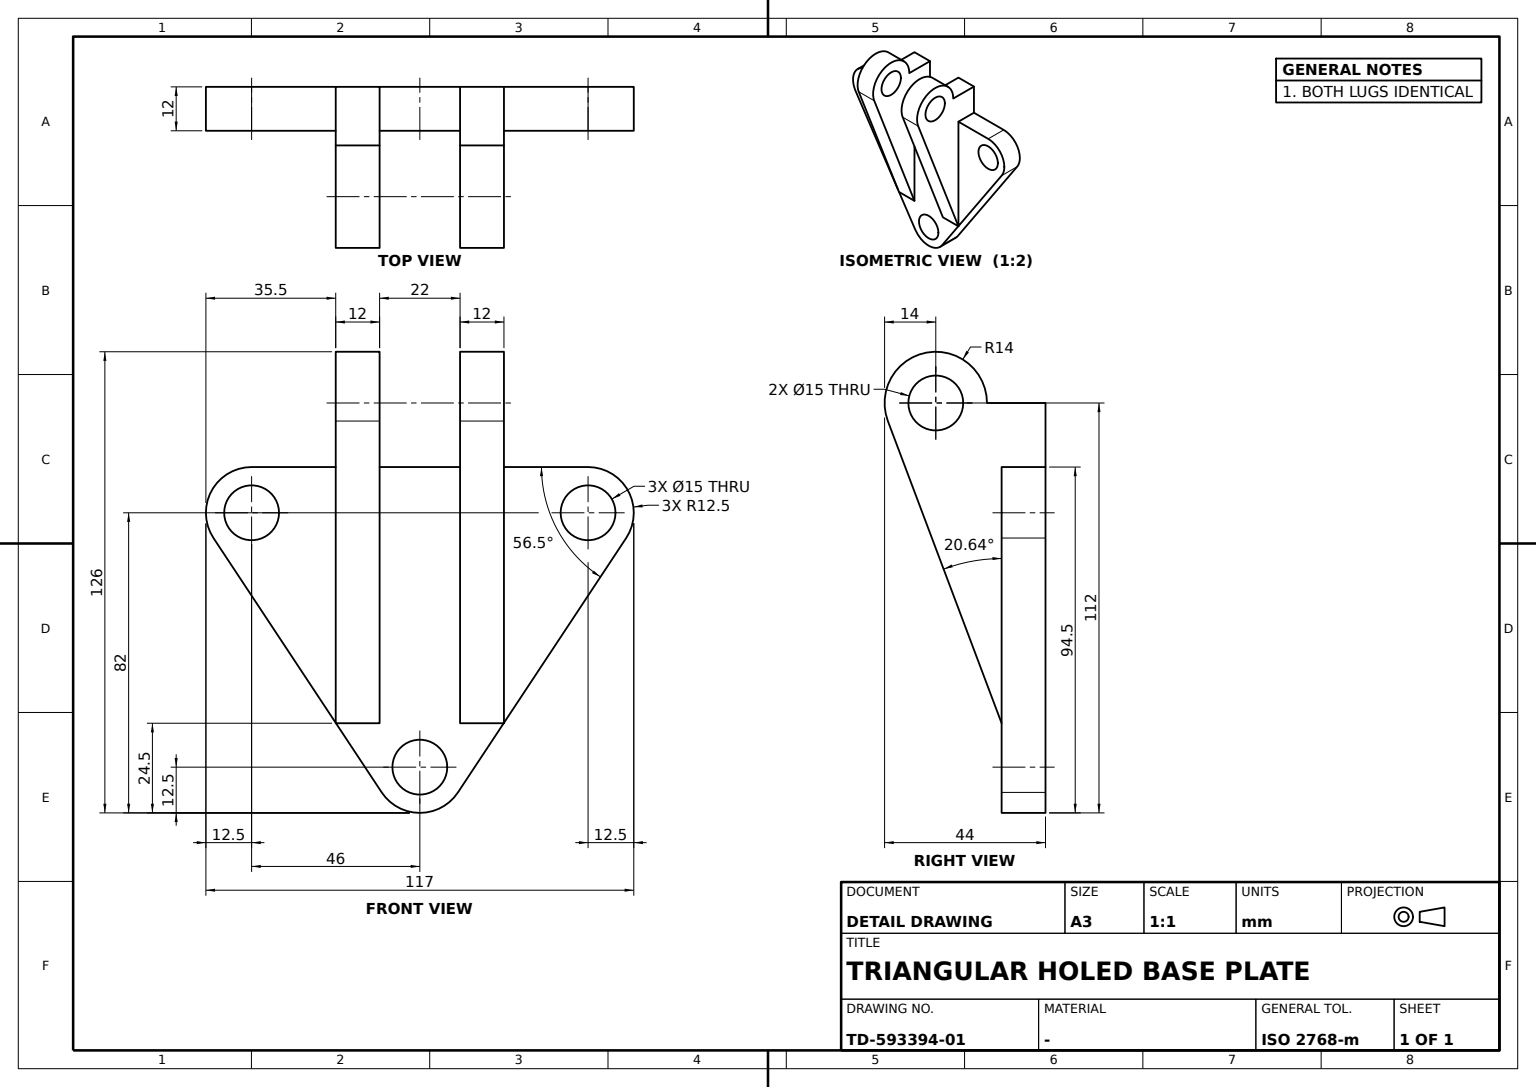
ISO-10303-21;
HEADER;
FILE_DESCRIPTION((''),'2;1');
FILE_NAME('','',(''),(''),'','','');
FILE_SCHEMA(('AUTOMOTIVE_DESIGN'));
ENDSEC;
DATA;
#1=APPLICATION_CONTEXT('');
#2=PRODUCT_CONTEXT('',#1,'mechanical');
#3=PRODUCT('','','',(#2));
#4=PRODUCT_DEFINITION_FORMATION('','',#3);
#5=PRODUCT_DEFINITION_CONTEXT('',#1,'design');
#6=PRODUCT_DEFINITION('','',#4,#5);
#7=PRODUCT_DEFINITION_SHAPE('','',#6);
#8=(LENGTH_UNIT()NAMED_UNIT(*)SI_UNIT(.MILLI.,.METRE.));
#9=(NAMED_UNIT(*)PLANE_ANGLE_UNIT()SI_UNIT($,.RADIAN.));
#10=(NAMED_UNIT(*)SI_UNIT($,.STERADIAN.)SOLID_ANGLE_UNIT());
#11=UNCERTAINTY_MEASURE_WITH_UNIT(LENGTH_MEASURE(1.E-05),#8,'distance_accuracy_value','');
#12=(GEOMETRIC_REPRESENTATION_CONTEXT(3)GLOBAL_UNCERTAINTY_ASSIGNED_CONTEXT((#11))GLOBAL_UNIT_ASSIGNED_CONTEXT((#8,#9,#10))REPRESENTATION_CONTEXT('',''));
#13=CARTESIAN_POINT('',(37.5,-11.,30.));
#14=VERTEX_POINT('',#13);
#15=CARTESIAN_POINT('',(22.5,-11.,30.));
#16=VERTEX_POINT('',#15);
#17=CARTESIAN_POINT('',(30.,-11.,30.));
#18=DIRECTION('',(0.,1.,0.));
#19=DIRECTION('',(-1.,0.,0.));
#20=AXIS2_PLACEMENT_3D('',#17,#18,#19);
#21=CIRCLE('',#20,7.5);
#22=EDGE_CURVE('',#14,#16,#21,.T.);
#23=ORIENTED_EDGE('',*,*,#22,.F.);
#24=EDGE_CURVE('',#16,#14,#21,.T.);
#25=ORIENTED_EDGE('',*,*,#24,.F.);
#26=EDGE_LOOP('',(#23,#25));
#27=FACE_BOUND('',#26,.T.);
#28=CARTESIAN_POINT('',(12.,-11.,12.5));
#29=VERTEX_POINT('',#28);
#30=CARTESIAN_POINT('',(0.,-11.,12.5));
#31=VERTEX_POINT('',#30);
#32=CARTESIAN_POINT('',(6.,-11.,12.5));
#33=VECTOR('',#19,1000.);
#34=LINE('',#32,#33);
#35=EDGE_CURVE('',#29,#31,#34,.T.);
#36=ORIENTED_EDGE('',*,*,#35,.T.);
#37=CARTESIAN_POINT('',(0.,-11.,30.));
#38=VERTEX_POINT('',#37);
#39=CARTESIAN_POINT('',(0.,-11.,21.25));
#40=DIRECTION('',(0.,0.,1.));
#41=VECTOR('',#40,1000.);
#42=LINE('',#39,#41);
#43=EDGE_CURVE('',#31,#38,#42,.T.);
#44=ORIENTED_EDGE('',*,*,#43,.T.);
#45=CARTESIAN_POINT('',(16.,-11.,30.));
#46=VERTEX_POINT('',#45);
#47=CARTESIAN_POINT('',(8.,-11.,30.));
#48=DIRECTION('',(1.,0.,0.));
#49=VECTOR('',#48,1000.);
#50=LINE('',#47,#49);
#51=EDGE_CURVE('',#38,#46,#50,.T.);
#52=ORIENTED_EDGE('',*,*,#51,.T.);
#53=CARTESIAN_POINT('',(43.101317,-11.,25.064872));
#54=VERTEX_POINT('',#53);
#55=CIRCLE('',#20,14.);
#56=EDGE_CURVE('',#46,#54,#55,.T.);
#57=ORIENTED_EDGE('',*,*,#56,.T.);
#58=CARTESIAN_POINT('',(12.,-11.,-57.5));
#59=VERTEX_POINT('',#58);
#60=CARTESIAN_POINT('',(27.550659,-11.,-16.217564));
#61=DIRECTION('',(-0.35250915,0.,-0.935808367));
#62=VECTOR('',#61,1000.);
#63=LINE('',#60,#62);
#64=EDGE_CURVE('',#54,#59,#63,.T.);
#65=ORIENTED_EDGE('',*,*,#64,.T.);
#66=CARTESIAN_POINT('',(12.,-11.,-22.5));
#67=LINE('',#66,#41);
#68=EDGE_CURVE('',#59,#29,#67,.T.);
#69=ORIENTED_EDGE('',*,*,#68,.T.);
#70=EDGE_LOOP('',(#36,#44,#52,#57,#65,#69));
#71=FACE_OUTER_BOUND('',#70,.T.);
#72=CARTESIAN_POINT('',(0.,-11.,0.));
#73=AXIS2_PLACEMENT_3D('',#72,#18,#19);
#74=PLANE('',#73);
#75=ADVANCED_FACE('',(#27,#71),#74,.T.);
#76=CARTESIAN_POINT('',(0.,38.5,0.));
#77=VERTEX_POINT('',#76);
#78=CARTESIAN_POINT('',(0.,53.5,0.));
#79=VERTEX_POINT('',#78);
#80=CARTESIAN_POINT('',(0.,46.,0.));
#81=AXIS2_PLACEMENT_3D('',#80,#48,#18);
#82=CIRCLE('',#81,7.5);
#83=EDGE_CURVE('',#77,#79,#82,.T.);
#84=ORIENTED_EDGE('',*,*,#83,.F.);
#85=CARTESIAN_POINT('',(12.,38.5,0.));
#86=VERTEX_POINT('',#85);
#87=CARTESIAN_POINT('',(6.,38.5,0.));
#88=LINE('',#87,#49);
#89=EDGE_CURVE('',#77,#86,#88,.T.);
#90=ORIENTED_EDGE('',*,*,#89,.T.);
#91=CARTESIAN_POINT('',(12.,53.5,0.));
#92=VERTEX_POINT('',#91);
#93=CARTESIAN_POINT('',(12.,46.,0.));
#94=AXIS2_PLACEMENT_3D('',#93,#48,#18);
#95=CIRCLE('',#94,7.5);
#96=EDGE_CURVE('',#86,#92,#95,.T.);
#97=ORIENTED_EDGE('',*,*,#96,.T.);
#98=CARTESIAN_POINT('',(6.,53.5,0.));
#99=LINE('',#98,#49);
#100=EDGE_CURVE('',#79,#92,#99,.T.);
#101=ORIENTED_EDGE('',*,*,#100,.F.);
#102=EDGE_LOOP('',(#84,#90,#97,#101));
#103=FACE_OUTER_BOUND('',#102,.T.);
#104=CARTESIAN_POINT('',(6.,46.,0.));
#105=AXIS2_PLACEMENT_3D('',#104,#19,#18);
#106=CYLINDRICAL_SURFACE('',#105,7.5);
#107=ADVANCED_FACE('',(#103),#106,.F.);
#108=CARTESIAN_POINT('',(0.,11.,30.));
#109=VERTEX_POINT('',#108);
#110=CARTESIAN_POINT('',(16.,11.,30.));
#111=VERTEX_POINT('',#110);
#112=CARTESIAN_POINT('',(8.,11.,30.));
#113=LINE('',#112,#49);
#114=EDGE_CURVE('',#109,#111,#113,.T.);
#115=ORIENTED_EDGE('',*,*,#114,.T.);
#116=CARTESIAN_POINT('',(16.,23.,30.));
#117=VERTEX_POINT('',#116);
#118=CARTESIAN_POINT('',(16.,17.,30.));
#119=VECTOR('',#18,1000.);
#120=LINE('',#118,#119);
#121=EDGE_CURVE('',#111,#117,#120,.T.);
#122=ORIENTED_EDGE('',*,*,#121,.T.);
#123=CARTESIAN_POINT('',(0.,23.,30.));
#124=VERTEX_POINT('',#123);
#125=CARTESIAN_POINT('',(8.,23.,30.));
#126=LINE('',#125,#49);
#127=EDGE_CURVE('',#124,#117,#126,.T.);
#128=ORIENTED_EDGE('',*,*,#127,.F.);
#129=CARTESIAN_POINT('',(0.,17.,30.));
#130=LINE('',#129,#119);
#131=EDGE_CURVE('',#109,#124,#130,.T.);
#132=ORIENTED_EDGE('',*,*,#131,.F.);
#133=EDGE_LOOP('',(#115,#122,#128,#132));
#134=FACE_OUTER_BOUND('',#133,.T.);
#135=CARTESIAN_POINT('',(16.,0.,30.));
#136=DIRECTION('',(0.,0.,-1.));
#137=AXIS2_PLACEMENT_3D('',#135,#136,#19);
#138=PLANE('',#137);
#139=ADVANCED_FACE('',(#134),#138,.F.);
#140=CARTESIAN_POINT('',(0.,-7.5,-69.5));
#141=VERTEX_POINT('',#140);
#142=CARTESIAN_POINT('',(12.,-7.5,-69.5));
#143=VERTEX_POINT('',#142);
#144=CARTESIAN_POINT('',(6.,-7.5,-69.5));
#145=LINE('',#144,#49);
#146=EDGE_CURVE('',#141,#143,#145,.T.);
#147=ORIENTED_EDGE('',*,*,#146,.F.);
#148=CARTESIAN_POINT('',(0.,7.5,-69.5));
#149=VERTEX_POINT('',#148);
#150=CARTESIAN_POINT('',(0.,0.,-69.5));
#151=AXIS2_PLACEMENT_3D('',#150,#48,#18);
#152=CIRCLE('',#151,7.5);
#153=EDGE_CURVE('',#149,#141,#152,.T.);
#154=ORIENTED_EDGE('',*,*,#153,.F.);
#155=CARTESIAN_POINT('',(12.,7.5,-69.5));
#156=VERTEX_POINT('',#155);
#157=CARTESIAN_POINT('',(6.,7.5,-69.5));
#158=LINE('',#157,#49);
#159=EDGE_CURVE('',#149,#156,#158,.T.);
#160=ORIENTED_EDGE('',*,*,#159,.T.);
#161=CARTESIAN_POINT('',(12.,0.,-69.5));
#162=AXIS2_PLACEMENT_3D('',#161,#48,#18);
#163=CIRCLE('',#162,7.5);
#164=EDGE_CURVE('',#156,#143,#163,.T.);
#165=ORIENTED_EDGE('',*,*,#164,.T.);
#166=EDGE_LOOP('',(#147,#154,#160,#165));
#167=FACE_OUTER_BOUND('',#166,.T.);
#168=CARTESIAN_POINT('',(6.,0.,-69.5));
#169=AXIS2_PLACEMENT_3D('',#168,#19,#18);
#170=CYLINDRICAL_SURFACE('',#169,7.5);
#171=ADVANCED_FACE('',(#167),#170,.F.);
#172=CARTESIAN_POINT('',(37.5,11.,30.));
#173=VERTEX_POINT('',#172);
#174=CARTESIAN_POINT('',(37.5,23.,30.));
#175=VERTEX_POINT('',#174);
#176=CARTESIAN_POINT('',(37.5,17.,30.));
#177=LINE('',#176,#119);
#178=EDGE_CURVE('',#173,#175,#177,.T.);
#179=ORIENTED_EDGE('',*,*,#178,.T.);
#180=CARTESIAN_POINT('',(22.5,23.,30.));
#181=VERTEX_POINT('',#180);
#182=CARTESIAN_POINT('',(30.,23.,30.));
#183=AXIS2_PLACEMENT_3D('',#182,#18,#19);
#184=CIRCLE('',#183,7.5);
#185=EDGE_CURVE('',#175,#181,#184,.T.);
#186=ORIENTED_EDGE('',*,*,#185,.T.);
#187=CARTESIAN_POINT('',(22.5,11.,30.));
#188=VERTEX_POINT('',#187);
#189=CARTESIAN_POINT('',(22.5,17.,30.));
#190=LINE('',#189,#119);
#191=EDGE_CURVE('',#188,#181,#190,.T.);
#192=ORIENTED_EDGE('',*,*,#191,.F.);
#193=CARTESIAN_POINT('',(30.,11.,30.));
#194=AXIS2_PLACEMENT_3D('',#193,#18,#19);
#195=CIRCLE('',#194,7.5);
#196=EDGE_CURVE('',#173,#188,#195,.T.);
#197=ORIENTED_EDGE('',*,*,#196,.F.);
#198=EDGE_LOOP('',(#179,#186,#192,#197));
#199=FACE_OUTER_BOUND('',#198,.T.);
#200=CARTESIAN_POINT('',(30.,17.,30.));
#201=DIRECTION('',(0.,-1.,0.));
#202=AXIS2_PLACEMENT_3D('',#200,#201,#19);
#203=CYLINDRICAL_SURFACE('',#202,7.5);
#204=ADVANCED_FACE('',(#199),#203,.F.);
#205=CARTESIAN_POINT('',(0.,11.,12.5));
#206=VERTEX_POINT('',#205);
#207=CARTESIAN_POINT('',(0.,0.,12.5));
#208=VECTOR('',#201,1000.);
#209=LINE('',#207,#208);
#210=EDGE_CURVE('',#206,#31,#209,.T.);
#211=ORIENTED_EDGE('',*,*,#210,.T.);
#212=ORIENTED_EDGE('',*,*,#35,.F.);
#213=CARTESIAN_POINT('',(12.,11.,12.5));
#214=VERTEX_POINT('',#213);
#215=CARTESIAN_POINT('',(12.,0.,12.5));
#216=LINE('',#215,#208);
#217=EDGE_CURVE('',#214,#29,#216,.T.);
#218=ORIENTED_EDGE('',*,*,#217,.F.);
#219=CARTESIAN_POINT('',(6.,11.,12.5));
#220=LINE('',#219,#33);
#221=EDGE_CURVE('',#214,#206,#220,.T.);
#222=ORIENTED_EDGE('',*,*,#221,.T.);
#223=EDGE_LOOP('',(#211,#212,#218,#222));
#224=FACE_OUTER_BOUND('',#223,.T.);
#225=CARTESIAN_POINT('',(0.,-46.,12.5));
#226=AXIS2_PLACEMENT_3D('',#225,#136,#18);
#227=PLANE('',#226);
#228=ADVANCED_FACE('',(#224),#227,.F.);
#229=CARTESIAN_POINT('',(12.,56.423645,-6.899103));
#230=VERTEX_POINT('',#229);
#231=CARTESIAN_POINT('',(12.,23.,-57.397871));
#232=VERTEX_POINT('',#231);
#233=CARTESIAN_POINT('',(12.,39.711823,-32.148487));
#234=DIRECTION('',(0.,-0.551928254,-0.833891601));
#235=VECTOR('',#234,1000.);
#236=LINE('',#233,#235);
#237=EDGE_CURVE('',#230,#232,#236,.T.);
#238=ORIENTED_EDGE('',*,*,#237,.T.);
#239=CARTESIAN_POINT('',(12.,22.932404,-57.5));
#240=VERTEX_POINT('',#239);
#241=CARTESIAN_POINT('',(12.,22.966202,-57.448936));
#242=LINE('',#241,#235);
#243=EDGE_CURVE('',#232,#240,#242,.T.);
#244=ORIENTED_EDGE('',*,*,#243,.T.);
#245=CARTESIAN_POINT('',(12.,10.423645,-76.399103));
#246=VERTEX_POINT('',#245);
#247=CARTESIAN_POINT('',(12.,16.678024,-66.949552));
#248=LINE('',#247,#235);
#249=EDGE_CURVE('',#240,#246,#248,.T.);
#250=ORIENTED_EDGE('',*,*,#249,.T.);
#251=CARTESIAN_POINT('',(0.,10.423645,-76.399103));
#252=VERTEX_POINT('',#251);
#253=CARTESIAN_POINT('',(6.,10.423645,-76.399103));
#254=LINE('',#253,#49);
#255=EDGE_CURVE('',#252,#246,#254,.T.);
#256=ORIENTED_EDGE('',*,*,#255,.F.);
#257=CARTESIAN_POINT('',(0.,56.423645,-6.899103));
#258=VERTEX_POINT('',#257);
#259=CARTESIAN_POINT('',(0.,33.423645,-41.649103));
#260=LINE('',#259,#235);
#261=EDGE_CURVE('',#258,#252,#260,.T.);
#262=ORIENTED_EDGE('',*,*,#261,.F.);
#263=CARTESIAN_POINT('',(6.,56.423645,-6.899103));
#264=LINE('',#263,#49);
#265=EDGE_CURVE('',#258,#230,#264,.T.);
#266=ORIENTED_EDGE('',*,*,#265,.T.);
#267=EDGE_LOOP('',(#238,#244,#250,#256,#262,#266));
#268=FACE_OUTER_BOUND('',#267,.T.);
#269=DIRECTION('',(0.,0.833891601,-0.551928254));
#270=DIRECTION('',(0.,0.551928254,0.833891601));
#271=AXIS2_PLACEMENT_3D('',#251,#269,#270);
#272=PLANE('',#271);
#273=ADVANCED_FACE('',(#268),#272,.T.);
#274=CARTESIAN_POINT('',(0.,58.5,0.));
#275=VERTEX_POINT('',#274);
#276=CIRCLE('',#81,12.5);
#277=EDGE_CURVE('',#258,#275,#276,.T.);
#278=ORIENTED_EDGE('',*,*,#277,.T.);
#279=CARTESIAN_POINT('',(12.,58.5,0.));
#280=VERTEX_POINT('',#279);
#281=CARTESIAN_POINT('',(6.,58.5,0.));
#282=LINE('',#281,#33);
#283=EDGE_CURVE('',#280,#275,#282,.T.);
#284=ORIENTED_EDGE('',*,*,#283,.F.);
#285=CIRCLE('',#94,12.5);
#286=EDGE_CURVE('',#230,#280,#285,.T.);
#287=ORIENTED_EDGE('',*,*,#286,.F.);
#288=ORIENTED_EDGE('',*,*,#265,.F.);
#289=EDGE_LOOP('',(#278,#284,#287,#288));
#290=FACE_OUTER_BOUND('',#289,.T.);
#291=CYLINDRICAL_SURFACE('',#105,12.5);
#292=ADVANCED_FACE('',(#290),#291,.T.);
#293=CARTESIAN_POINT('',(43.101317,-23.,25.064872));
#294=VERTEX_POINT('',#293);
#295=CARTESIAN_POINT('',(43.101317,17.,25.064872));
#296=LINE('',#295,#208);
#297=EDGE_CURVE('',#54,#294,#296,.T.);
#298=ORIENTED_EDGE('',*,*,#297,.F.);
#299=ORIENTED_EDGE('',*,*,#56,.F.);
#300=CARTESIAN_POINT('',(16.,-23.,30.));
#301=VERTEX_POINT('',#300);
#302=LINE('',#118,#208);
#303=EDGE_CURVE('',#46,#301,#302,.T.);
#304=ORIENTED_EDGE('',*,*,#303,.T.);
#305=CARTESIAN_POINT('',(30.,-23.,30.));
#306=AXIS2_PLACEMENT_3D('',#305,#18,#19);
#307=CIRCLE('',#306,14.);
#308=EDGE_CURVE('',#301,#294,#307,.T.);
#309=ORIENTED_EDGE('',*,*,#308,.T.);
#310=EDGE_LOOP('',(#298,#299,#304,#309));
#311=FACE_OUTER_BOUND('',#310,.T.);
#312=CYLINDRICAL_SURFACE('',#202,14.);
#313=ADVANCED_FACE('',(#311),#312,.T.);
#314=CARTESIAN_POINT('',(43.101317,23.,25.064872));
#315=VERTEX_POINT('',#314);
#316=CARTESIAN_POINT('',(12.,23.,-57.5));
#317=VERTEX_POINT('',#316);
#318=CARTESIAN_POINT('',(27.550659,23.,-16.217564));
#319=LINE('',#318,#62);
#320=EDGE_CURVE('',#315,#317,#319,.T.);
#321=ORIENTED_EDGE('',*,*,#320,.F.);
#322=CARTESIAN_POINT('',(43.101317,11.,25.064872));
#323=VERTEX_POINT('',#322);
#324=LINE('',#295,#119);
#325=EDGE_CURVE('',#323,#315,#324,.T.);
#326=ORIENTED_EDGE('',*,*,#325,.F.);
#327=CARTESIAN_POINT('',(12.,11.,-57.5));
#328=VERTEX_POINT('',#327);
#329=CARTESIAN_POINT('',(27.550659,11.,-16.217564));
#330=LINE('',#329,#62);
#331=EDGE_CURVE('',#323,#328,#330,.T.);
#332=ORIENTED_EDGE('',*,*,#331,.T.);
#333=CARTESIAN_POINT('',(12.,16.966202,-57.5));
#334=LINE('',#333,#119);
#335=EDGE_CURVE('',#328,#240,#334,.T.);
#336=ORIENTED_EDGE('',*,*,#335,.T.);
#337=CARTESIAN_POINT('',(12.,22.966202,-57.5));
#338=LINE('',#337,#119);
#339=EDGE_CURVE('',#240,#317,#338,.T.);
#340=ORIENTED_EDGE('',*,*,#339,.T.);
#341=EDGE_LOOP('',(#321,#326,#332,#336,#340));
#342=FACE_OUTER_BOUND('',#341,.T.);
#343=CARTESIAN_POINT('',(43.101317,0.,25.064872));
#344=DIRECTION('',(0.935808367,0.,-0.35250915));
#345=AXIS2_PLACEMENT_3D('',#343,#344,#61);
#346=PLANE('',#345);
#347=ADVANCED_FACE('',(#342),#346,.T.);
#348=EDGE_CURVE('',#92,#86,#95,.T.);
#349=ORIENTED_EDGE('',*,*,#348,.F.);
#350=ORIENTED_EDGE('',*,*,#96,.F.);
#351=EDGE_LOOP('',(#349,#350));
#352=FACE_BOUND('',#351,.T.);
#353=ORIENTED_EDGE('',*,*,#286,.T.);
#354=CARTESIAN_POINT('',(12.,46.,12.5));
#355=VERTEX_POINT('',#354);
#356=EDGE_CURVE('',#280,#355,#285,.T.);
#357=ORIENTED_EDGE('',*,*,#356,.T.);
#358=CARTESIAN_POINT('',(12.,23.,12.5));
#359=VERTEX_POINT('',#358);
#360=CARTESIAN_POINT('',(12.,34.5,12.5));
#361=LINE('',#360,#208);
#362=EDGE_CURVE('',#355,#359,#361,.T.);
#363=ORIENTED_EDGE('',*,*,#362,.T.);
#364=CARTESIAN_POINT('',(12.,23.,-22.448936));
#365=LINE('',#364,#41);
#366=EDGE_CURVE('',#232,#359,#365,.T.);
#367=ORIENTED_EDGE('',*,*,#366,.F.);
#368=ORIENTED_EDGE('',*,*,#237,.F.);
#369=EDGE_LOOP('',(#353,#357,#363,#367,#368));
#370=FACE_OUTER_BOUND('',#369,.T.);
#371=CARTESIAN_POINT('',(12.,0.,0.));
#372=AXIS2_PLACEMENT_3D('',#371,#48,#18);
#373=PLANE('',#372);
#374=ADVANCED_FACE('',(#352,#370),#373,.T.);
#375=CARTESIAN_POINT('',(0.,46.,12.5));
#376=VERTEX_POINT('',#375);
#377=CARTESIAN_POINT('',(0.,23.,12.5));
#378=VERTEX_POINT('',#377);
#379=CARTESIAN_POINT('',(0.,34.5,12.5));
#380=LINE('',#379,#208);
#381=EDGE_CURVE('',#376,#378,#380,.T.);
#382=ORIENTED_EDGE('',*,*,#381,.T.);
#383=CARTESIAN_POINT('',(6.,23.,12.5));
#384=LINE('',#383,#33);
#385=EDGE_CURVE('',#359,#378,#384,.T.);
#386=ORIENTED_EDGE('',*,*,#385,.F.);
#387=ORIENTED_EDGE('',*,*,#362,.F.);
#388=CARTESIAN_POINT('',(6.,46.,12.5));
#389=LINE('',#388,#49);
#390=EDGE_CURVE('',#376,#355,#389,.T.);
#391=ORIENTED_EDGE('',*,*,#390,.F.);
#392=EDGE_LOOP('',(#382,#386,#387,#391));
#393=FACE_OUTER_BOUND('',#392,.T.);
#394=ADVANCED_FACE('',(#393),#227,.F.);
#395=CARTESIAN_POINT('',(12.,23.,-57.448936));
#396=LINE('',#395,#41);
#397=EDGE_CURVE('',#317,#232,#396,.T.);
#398=ORIENTED_EDGE('',*,*,#397,.F.);
#399=ORIENTED_EDGE('',*,*,#339,.F.);
#400=ORIENTED_EDGE('',*,*,#243,.F.);
#401=EDGE_LOOP('',(#398,#399,#400));
#402=FACE_OUTER_BOUND('',#401,.T.);
#403=ADVANCED_FACE('',(#402),#373,.F.);
#404=CARTESIAN_POINT('',(0.,-38.5,0.));
#405=VERTEX_POINT('',#404);
#406=CARTESIAN_POINT('',(12.,-38.5,0.));
#407=VERTEX_POINT('',#406);
#408=CARTESIAN_POINT('',(6.,-38.5,0.));
#409=LINE('',#408,#49);
#410=EDGE_CURVE('',#405,#407,#409,.T.);
#411=ORIENTED_EDGE('',*,*,#410,.F.);
#412=CARTESIAN_POINT('',(0.,-53.5,0.));
#413=VERTEX_POINT('',#412);
#414=CARTESIAN_POINT('',(0.,-46.,0.));
#415=AXIS2_PLACEMENT_3D('',#414,#48,#18);
#416=CIRCLE('',#415,7.5);
#417=EDGE_CURVE('',#413,#405,#416,.T.);
#418=ORIENTED_EDGE('',*,*,#417,.F.);
#419=CARTESIAN_POINT('',(12.,-53.5,0.));
#420=VERTEX_POINT('',#419);
#421=CARTESIAN_POINT('',(6.,-53.5,0.));
#422=LINE('',#421,#49);
#423=EDGE_CURVE('',#413,#420,#422,.T.);
#424=ORIENTED_EDGE('',*,*,#423,.T.);
#425=CARTESIAN_POINT('',(12.,-46.,0.));
#426=AXIS2_PLACEMENT_3D('',#425,#48,#18);
#427=CIRCLE('',#426,7.5);
#428=EDGE_CURVE('',#420,#407,#427,.T.);
#429=ORIENTED_EDGE('',*,*,#428,.T.);
#430=EDGE_LOOP('',(#411,#418,#424,#429));
#431=FACE_OUTER_BOUND('',#430,.T.);
#432=CARTESIAN_POINT('',(6.,-46.,0.));
#433=AXIS2_PLACEMENT_3D('',#432,#19,#18);
#434=CYLINDRICAL_SURFACE('',#433,7.5);
#435=ADVANCED_FACE('',(#431),#434,.F.);
#436=ORIENTED_EDGE('',*,*,#114,.F.);
#437=CARTESIAN_POINT('',(0.,11.,21.25));
#438=LINE('',#437,#41);
#439=EDGE_CURVE('',#206,#109,#438,.T.);
#440=ORIENTED_EDGE('',*,*,#439,.F.);
#441=ORIENTED_EDGE('',*,*,#221,.F.);
#442=CARTESIAN_POINT('',(12.,11.,-22.5));
#443=LINE('',#442,#41);
#444=EDGE_CURVE('',#328,#214,#443,.T.);
#445=ORIENTED_EDGE('',*,*,#444,.F.);
#446=ORIENTED_EDGE('',*,*,#331,.F.);
#447=CIRCLE('',#194,14.);
#448=EDGE_CURVE('',#111,#323,#447,.T.);
#449=ORIENTED_EDGE('',*,*,#448,.F.);
#450=EDGE_LOOP('',(#436,#440,#441,#445,#446,#449));
#451=FACE_OUTER_BOUND('',#450,.T.);
#452=EDGE_CURVE('',#188,#173,#195,.T.);
#453=ORIENTED_EDGE('',*,*,#452,.T.);
#454=ORIENTED_EDGE('',*,*,#196,.T.);
#455=EDGE_LOOP('',(#453,#454));
#456=FACE_BOUND('',#455,.T.);
#457=CARTESIAN_POINT('',(0.,11.,0.));
#458=AXIS2_PLACEMENT_3D('',#457,#18,#19);
#459=PLANE('',#458);
#460=ADVANCED_FACE('',(#451,#456),#459,.F.);
#461=CARTESIAN_POINT('',(0.,-10.423645,-76.399103));
#462=VERTEX_POINT('',#461);
#463=CARTESIAN_POINT('',(12.,-10.423645,-76.399103));
#464=VERTEX_POINT('',#463);
#465=CARTESIAN_POINT('',(6.,-10.423645,-76.399103));
#466=LINE('',#465,#49);
#467=EDGE_CURVE('',#462,#464,#466,.T.);
#468=ORIENTED_EDGE('',*,*,#467,.F.);
#469=CIRCLE('',#151,12.5);
#470=EDGE_CURVE('',#462,#252,#469,.T.);
#471=ORIENTED_EDGE('',*,*,#470,.T.);
#472=ORIENTED_EDGE('',*,*,#255,.T.);
#473=CIRCLE('',#162,12.5);
#474=EDGE_CURVE('',#464,#246,#473,.T.);
#475=ORIENTED_EDGE('',*,*,#474,.F.);
#476=EDGE_LOOP('',(#468,#471,#472,#475));
#477=FACE_OUTER_BOUND('',#476,.T.);
#478=CYLINDRICAL_SURFACE('',#169,12.5);
#479=ADVANCED_FACE('',(#477),#478,.T.);
#480=ORIENTED_EDGE('',*,*,#83,.T.);
#481=EDGE_CURVE('',#79,#77,#82,.T.);
#482=ORIENTED_EDGE('',*,*,#481,.T.);
#483=EDGE_LOOP('',(#480,#482));
#484=FACE_BOUND('',#483,.T.);
#485=ORIENTED_EDGE('',*,*,#470,.F.);
#486=CARTESIAN_POINT('',(0.,-56.423645,-6.899103));
#487=VERTEX_POINT('',#486);
#488=CARTESIAN_POINT('',(0.,-33.423645,-41.649103));
#489=DIRECTION('',(0.,0.551928254,-0.833891601));
#490=VECTOR('',#489,1000.);
#491=LINE('',#488,#490);
#492=EDGE_CURVE('',#487,#462,#491,.T.);
#493=ORIENTED_EDGE('',*,*,#492,.F.);
#494=VERTEX_POINT('',#225);
#495=CIRCLE('',#415,12.5);
#496=EDGE_CURVE('',#494,#487,#495,.T.);
#497=ORIENTED_EDGE('',*,*,#496,.F.);
#498=CARTESIAN_POINT('',(0.,-23.,12.5));
#499=VERTEX_POINT('',#498);
#500=CARTESIAN_POINT('',(0.,-34.5,12.5));
#501=LINE('',#500,#208);
#502=EDGE_CURVE('',#499,#494,#501,.T.);
#503=ORIENTED_EDGE('',*,*,#502,.F.);
#504=CARTESIAN_POINT('',(0.,-23.,30.));
#505=VERTEX_POINT('',#504);
#506=CARTESIAN_POINT('',(0.,-23.,21.25));
#507=LINE('',#506,#41);
#508=EDGE_CURVE('',#499,#505,#507,.T.);
#509=ORIENTED_EDGE('',*,*,#508,.T.);
#510=CARTESIAN_POINT('',(0.,-17.,30.));
#511=LINE('',#510,#208);
#512=EDGE_CURVE('',#38,#505,#511,.T.);
#513=ORIENTED_EDGE('',*,*,#512,.F.);
#514=ORIENTED_EDGE('',*,*,#43,.F.);
#515=ORIENTED_EDGE('',*,*,#210,.F.);
#516=ORIENTED_EDGE('',*,*,#439,.T.);
#517=ORIENTED_EDGE('',*,*,#131,.T.);
#518=CARTESIAN_POINT('',(0.,23.,21.25));
#519=LINE('',#518,#41);
#520=EDGE_CURVE('',#378,#124,#519,.T.);
#521=ORIENTED_EDGE('',*,*,#520,.F.);
#522=ORIENTED_EDGE('',*,*,#381,.F.);
#523=EDGE_CURVE('',#275,#376,#276,.T.);
#524=ORIENTED_EDGE('',*,*,#523,.F.);
#525=ORIENTED_EDGE('',*,*,#277,.F.);
#526=ORIENTED_EDGE('',*,*,#261,.T.);
#527=EDGE_LOOP('',(#485,#493,#497,#503,#509,#513,#514,#515,#516,#517,#521,#522,#524,#525,#526));
#528=FACE_OUTER_BOUND('',#527,.T.);
#529=ORIENTED_EDGE('',*,*,#153,.T.);
#530=EDGE_CURVE('',#141,#149,#152,.T.);
#531=ORIENTED_EDGE('',*,*,#530,.T.);
#532=EDGE_LOOP('',(#529,#531));
#533=FACE_BOUND('',#532,.T.);
#534=EDGE_CURVE('',#405,#413,#416,.T.);
#535=ORIENTED_EDGE('',*,*,#534,.T.);
#536=ORIENTED_EDGE('',*,*,#417,.T.);
#537=EDGE_LOOP('',(#535,#536));
#538=FACE_BOUND('',#537,.T.);
#539=CARTESIAN_POINT('',(0.,0.,0.));
#540=AXIS2_PLACEMENT_3D('',#539,#48,#18);
#541=PLANE('',#540);
#542=ADVANCED_FACE('',(#484,#528,#533,#538),#541,.F.);
#543=ORIENTED_EDGE('',*,*,#283,.T.);
#544=ORIENTED_EDGE('',*,*,#523,.T.);
#545=ORIENTED_EDGE('',*,*,#390,.T.);
#546=ORIENTED_EDGE('',*,*,#356,.F.);
#547=EDGE_LOOP('',(#543,#544,#545,#546));
#548=FACE_OUTER_BOUND('',#547,.T.);
#549=ADVANCED_FACE('',(#548),#291,.T.);
#550=ORIENTED_EDGE('',*,*,#325,.T.);
#551=CIRCLE('',#183,14.);
#552=EDGE_CURVE('',#117,#315,#551,.T.);
#553=ORIENTED_EDGE('',*,*,#552,.F.);
#554=ORIENTED_EDGE('',*,*,#121,.F.);
#555=ORIENTED_EDGE('',*,*,#448,.T.);
#556=EDGE_LOOP('',(#550,#553,#554,#555));
#557=FACE_OUTER_BOUND('',#556,.T.);
#558=ADVANCED_FACE('',(#557),#312,.T.);
#559=ORIENTED_EDGE('',*,*,#481,.F.);
#560=ORIENTED_EDGE('',*,*,#100,.T.);
#561=ORIENTED_EDGE('',*,*,#348,.T.);
#562=ORIENTED_EDGE('',*,*,#89,.F.);
#563=EDGE_LOOP('',(#559,#560,#561,#562));
#564=FACE_OUTER_BOUND('',#563,.T.);
#565=ADVANCED_FACE('',(#564),#106,.F.);
#566=ORIENTED_EDGE('',*,*,#496,.T.);
#567=CARTESIAN_POINT('',(12.,-56.423645,-6.899103));
#568=VERTEX_POINT('',#567);
#569=CARTESIAN_POINT('',(6.,-56.423645,-6.899103));
#570=LINE('',#569,#49);
#571=EDGE_CURVE('',#487,#568,#570,.T.);
#572=ORIENTED_EDGE('',*,*,#571,.T.);
#573=CARTESIAN_POINT('',(12.,-46.,12.5));
#574=VERTEX_POINT('',#573);
#575=CIRCLE('',#426,12.5);
#576=EDGE_CURVE('',#574,#568,#575,.T.);
#577=ORIENTED_EDGE('',*,*,#576,.F.);
#578=CARTESIAN_POINT('',(6.,-46.,12.5));
#579=LINE('',#578,#49);
#580=EDGE_CURVE('',#494,#574,#579,.T.);
#581=ORIENTED_EDGE('',*,*,#580,.F.);
#582=EDGE_LOOP('',(#566,#572,#577,#581));
#583=FACE_OUTER_BOUND('',#582,.T.);
#584=CYLINDRICAL_SURFACE('',#433,12.5);
#585=ADVANCED_FACE('',(#583),#584,.T.);
#586=ORIENTED_EDGE('',*,*,#423,.F.);
#587=ORIENTED_EDGE('',*,*,#534,.F.);
#588=ORIENTED_EDGE('',*,*,#410,.T.);
#589=EDGE_CURVE('',#407,#420,#427,.T.);
#590=ORIENTED_EDGE('',*,*,#589,.T.);
#591=EDGE_LOOP('',(#586,#587,#588,#590));
#592=FACE_OUTER_BOUND('',#591,.T.);
#593=ADVANCED_FACE('',(#592),#434,.F.);
#594=ORIENTED_EDGE('',*,*,#580,.T.);
#595=CARTESIAN_POINT('',(12.,-23.,12.5));
#596=VERTEX_POINT('',#595);
#597=CARTESIAN_POINT('',(12.,-34.5,12.5));
#598=LINE('',#597,#208);
#599=EDGE_CURVE('',#596,#574,#598,.T.);
#600=ORIENTED_EDGE('',*,*,#599,.F.);
#601=CARTESIAN_POINT('',(6.,-23.,12.5));
#602=LINE('',#601,#33);
#603=EDGE_CURVE('',#596,#499,#602,.T.);
#604=ORIENTED_EDGE('',*,*,#603,.T.);
#605=ORIENTED_EDGE('',*,*,#502,.T.);
#606=EDGE_LOOP('',(#594,#600,#604,#605));
#607=FACE_OUTER_BOUND('',#606,.T.);
#608=ADVANCED_FACE('',(#607),#227,.F.);
#609=ORIENTED_EDGE('',*,*,#576,.T.);
#610=CARTESIAN_POINT('',(12.,-23.,-57.397871));
#611=VERTEX_POINT('',#610);
#612=CARTESIAN_POINT('',(12.,-39.711823,-32.148487));
#613=LINE('',#612,#490);
#614=EDGE_CURVE('',#568,#611,#613,.T.);
#615=ORIENTED_EDGE('',*,*,#614,.T.);
#616=CARTESIAN_POINT('',(12.,-23.,-22.448936));
#617=LINE('',#616,#41);
#618=EDGE_CURVE('',#611,#596,#617,.T.);
#619=ORIENTED_EDGE('',*,*,#618,.T.);
#620=ORIENTED_EDGE('',*,*,#599,.T.);
#621=EDGE_LOOP('',(#609,#615,#619,#620));
#622=FACE_OUTER_BOUND('',#621,.T.);
#623=ORIENTED_EDGE('',*,*,#589,.F.);
#624=ORIENTED_EDGE('',*,*,#428,.F.);
#625=EDGE_LOOP('',(#623,#624));
#626=FACE_BOUND('',#625,.T.);
#627=ADVANCED_FACE('',(#622,#626),#373,.T.);
#628=CARTESIAN_POINT('',(22.5,-23.,30.));
#629=VERTEX_POINT('',#628);
#630=CARTESIAN_POINT('',(37.5,-23.,30.));
#631=VERTEX_POINT('',#630);
#632=CIRCLE('',#306,7.5);
#633=EDGE_CURVE('',#629,#631,#632,.T.);
#634=ORIENTED_EDGE('',*,*,#633,.F.);
#635=LINE('',#189,#208);
#636=EDGE_CURVE('',#16,#629,#635,.T.);
#637=ORIENTED_EDGE('',*,*,#636,.F.);
#638=ORIENTED_EDGE('',*,*,#24,.T.);
#639=LINE('',#176,#208);
#640=EDGE_CURVE('',#14,#631,#639,.T.);
#641=ORIENTED_EDGE('',*,*,#640,.T.);
#642=EDGE_LOOP('',(#634,#637,#638,#641));
#643=FACE_OUTER_BOUND('',#642,.T.);
#644=ADVANCED_FACE('',(#643),#203,.F.);
#645=ORIENTED_EDGE('',*,*,#178,.F.);
#646=ORIENTED_EDGE('',*,*,#452,.F.);
#647=ORIENTED_EDGE('',*,*,#191,.T.);
#648=EDGE_CURVE('',#181,#175,#184,.T.);
#649=ORIENTED_EDGE('',*,*,#648,.T.);
#650=EDGE_LOOP('',(#645,#646,#647,#649));
#651=FACE_OUTER_BOUND('',#650,.T.);
#652=ADVANCED_FACE('',(#651),#203,.F.);
#653=ORIENTED_EDGE('',*,*,#249,.F.);
#654=ORIENTED_EDGE('',*,*,#335,.F.);
#655=ORIENTED_EDGE('',*,*,#444,.T.);
#656=ORIENTED_EDGE('',*,*,#217,.T.);
#657=ORIENTED_EDGE('',*,*,#68,.F.);
#658=CARTESIAN_POINT('',(12.,-22.932404,-57.5));
#659=VERTEX_POINT('',#658);
#660=CARTESIAN_POINT('',(12.,-16.966202,-57.5));
#661=LINE('',#660,#208);
#662=EDGE_CURVE('',#59,#659,#661,.T.);
#663=ORIENTED_EDGE('',*,*,#662,.T.);
#664=CARTESIAN_POINT('',(12.,-16.678024,-66.949552));
#665=LINE('',#664,#490);
#666=EDGE_CURVE('',#659,#464,#665,.T.);
#667=ORIENTED_EDGE('',*,*,#666,.T.);
#668=ORIENTED_EDGE('',*,*,#474,.T.);
#669=EDGE_LOOP('',(#653,#654,#655,#656,#657,#663,#667,#668));
#670=FACE_OUTER_BOUND('',#669,.T.);
#671=EDGE_CURVE('',#143,#156,#163,.T.);
#672=ORIENTED_EDGE('',*,*,#671,.F.);
#673=ORIENTED_EDGE('',*,*,#164,.F.);
#674=EDGE_LOOP('',(#672,#673));
#675=FACE_BOUND('',#674,.T.);
#676=ADVANCED_FACE('',(#670,#675),#373,.T.);
#677=ORIENTED_EDGE('',*,*,#530,.F.);
#678=ORIENTED_EDGE('',*,*,#146,.T.);
#679=ORIENTED_EDGE('',*,*,#671,.T.);
#680=ORIENTED_EDGE('',*,*,#159,.F.);
#681=EDGE_LOOP('',(#677,#678,#679,#680));
#682=FACE_OUTER_BOUND('',#681,.T.);
#683=ADVANCED_FACE('',(#682),#170,.F.);
#684=ORIENTED_EDGE('',*,*,#492,.T.);
#685=ORIENTED_EDGE('',*,*,#467,.T.);
#686=ORIENTED_EDGE('',*,*,#666,.F.);
#687=CARTESIAN_POINT('',(12.,-22.966202,-57.448936));
#688=LINE('',#687,#490);
#689=EDGE_CURVE('',#611,#659,#688,.T.);
#690=ORIENTED_EDGE('',*,*,#689,.F.);
#691=ORIENTED_EDGE('',*,*,#614,.F.);
#692=ORIENTED_EDGE('',*,*,#571,.F.);
#693=EDGE_LOOP('',(#684,#685,#686,#690,#691,#692));
#694=FACE_OUTER_BOUND('',#693,.T.);
#695=DIRECTION('',(0.,-0.833891601,-0.551928254));
#696=AXIS2_PLACEMENT_3D('',#486,#695,#489);
#697=PLANE('',#696);
#698=ADVANCED_FACE('',(#694),#697,.T.);
#699=CARTESIAN_POINT('',(12.,-23.,-57.5));
#700=VERTEX_POINT('',#699);
#701=CARTESIAN_POINT('',(12.,-23.,-57.448936));
#702=LINE('',#701,#41);
#703=EDGE_CURVE('',#700,#611,#702,.T.);
#704=ORIENTED_EDGE('',*,*,#703,.T.);
#705=ORIENTED_EDGE('',*,*,#689,.T.);
#706=CARTESIAN_POINT('',(12.,-22.966202,-57.5));
#707=LINE('',#706,#208);
#708=EDGE_CURVE('',#659,#700,#707,.T.);
#709=ORIENTED_EDGE('',*,*,#708,.T.);
#710=EDGE_LOOP('',(#704,#705,#709));
#711=FACE_OUTER_BOUND('',#710,.T.);
#712=ADVANCED_FACE('',(#711),#373,.F.);
#713=ORIENTED_EDGE('',*,*,#648,.F.);
#714=ORIENTED_EDGE('',*,*,#185,.F.);
#715=EDGE_LOOP('',(#713,#714));
#716=FACE_BOUND('',#715,.T.);
#717=ORIENTED_EDGE('',*,*,#552,.T.);
#718=ORIENTED_EDGE('',*,*,#320,.T.);
#719=ORIENTED_EDGE('',*,*,#397,.T.);
#720=ORIENTED_EDGE('',*,*,#366,.T.);
#721=ORIENTED_EDGE('',*,*,#385,.T.);
#722=ORIENTED_EDGE('',*,*,#520,.T.);
#723=ORIENTED_EDGE('',*,*,#127,.T.);
#724=EDGE_LOOP('',(#717,#718,#719,#720,#721,#722,#723));
#725=FACE_OUTER_BOUND('',#724,.T.);
#726=CARTESIAN_POINT('',(0.,23.,0.));
#727=AXIS2_PLACEMENT_3D('',#726,#18,#19);
#728=PLANE('',#727);
#729=ADVANCED_FACE('',(#716,#725),#728,.T.);
#730=ORIENTED_EDGE('',*,*,#512,.T.);
#731=CARTESIAN_POINT('',(8.,-23.,30.));
#732=LINE('',#731,#49);
#733=EDGE_CURVE('',#505,#301,#732,.T.);
#734=ORIENTED_EDGE('',*,*,#733,.T.);
#735=ORIENTED_EDGE('',*,*,#303,.F.);
#736=ORIENTED_EDGE('',*,*,#51,.F.);
#737=EDGE_LOOP('',(#730,#734,#735,#736));
#738=FACE_OUTER_BOUND('',#737,.T.);
#739=ADVANCED_FACE('',(#738),#138,.F.);
#740=ORIENTED_EDGE('',*,*,#508,.F.);
#741=ORIENTED_EDGE('',*,*,#603,.F.);
#742=ORIENTED_EDGE('',*,*,#618,.F.);
#743=ORIENTED_EDGE('',*,*,#703,.F.);
#744=CARTESIAN_POINT('',(27.550659,-23.,-16.217564));
#745=LINE('',#744,#62);
#746=EDGE_CURVE('',#294,#700,#745,.T.);
#747=ORIENTED_EDGE('',*,*,#746,.F.);
#748=ORIENTED_EDGE('',*,*,#308,.F.);
#749=ORIENTED_EDGE('',*,*,#733,.F.);
#750=EDGE_LOOP('',(#740,#741,#742,#743,#747,#748,#749));
#751=FACE_OUTER_BOUND('',#750,.T.);
#752=EDGE_CURVE('',#631,#629,#632,.T.);
#753=ORIENTED_EDGE('',*,*,#752,.T.);
#754=ORIENTED_EDGE('',*,*,#633,.T.);
#755=EDGE_LOOP('',(#753,#754));
#756=FACE_BOUND('',#755,.T.);
#757=CARTESIAN_POINT('',(0.,-23.,0.));
#758=AXIS2_PLACEMENT_3D('',#757,#18,#19);
#759=PLANE('',#758);
#760=ADVANCED_FACE('',(#751,#756),#759,.F.);
#761=ORIENTED_EDGE('',*,*,#297,.T.);
#762=ORIENTED_EDGE('',*,*,#746,.T.);
#763=ORIENTED_EDGE('',*,*,#708,.F.);
#764=ORIENTED_EDGE('',*,*,#662,.F.);
#765=ORIENTED_EDGE('',*,*,#64,.F.);
#766=EDGE_LOOP('',(#761,#762,#763,#764,#765));
#767=FACE_OUTER_BOUND('',#766,.T.);
#768=ADVANCED_FACE('',(#767),#346,.T.);
#769=ORIENTED_EDGE('',*,*,#640,.F.);
#770=ORIENTED_EDGE('',*,*,#22,.T.);
#771=ORIENTED_EDGE('',*,*,#636,.T.);
#772=ORIENTED_EDGE('',*,*,#752,.F.);
#773=EDGE_LOOP('',(#769,#770,#771,#772));
#774=FACE_OUTER_BOUND('',#773,.T.);
#775=ADVANCED_FACE('',(#774),#203,.F.);
#776=CLOSED_SHELL('',(#75,#107,#139,#171,#204,#228,#273,#292,#313,#347,#374,#394,#403,#435,#460,#479,#542,#549,#558,#565,#585,#593,#608,#627,#644,#652,#676,#683,#698,#712,#729,#739,#760,#768,#775));
#777=MANIFOLD_SOLID_BREP('',#776);
#778=ADVANCED_BREP_SHAPE_REPRESENTATION('',(#777),#12);
#779=SHAPE_DEFINITION_REPRESENTATION(#7,#778);
ENDSEC;
END-ISO-10303-21;
